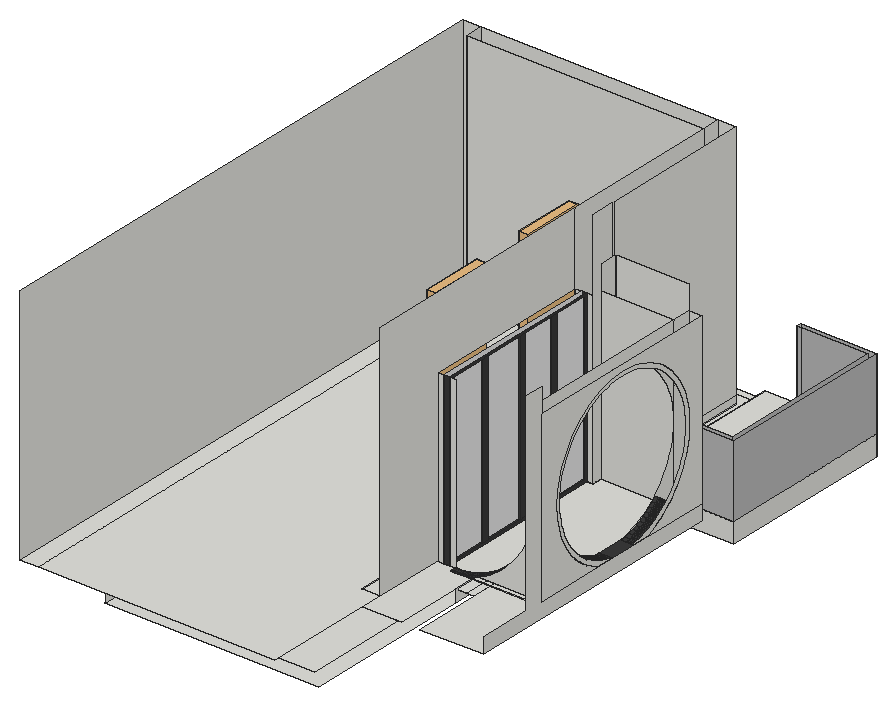
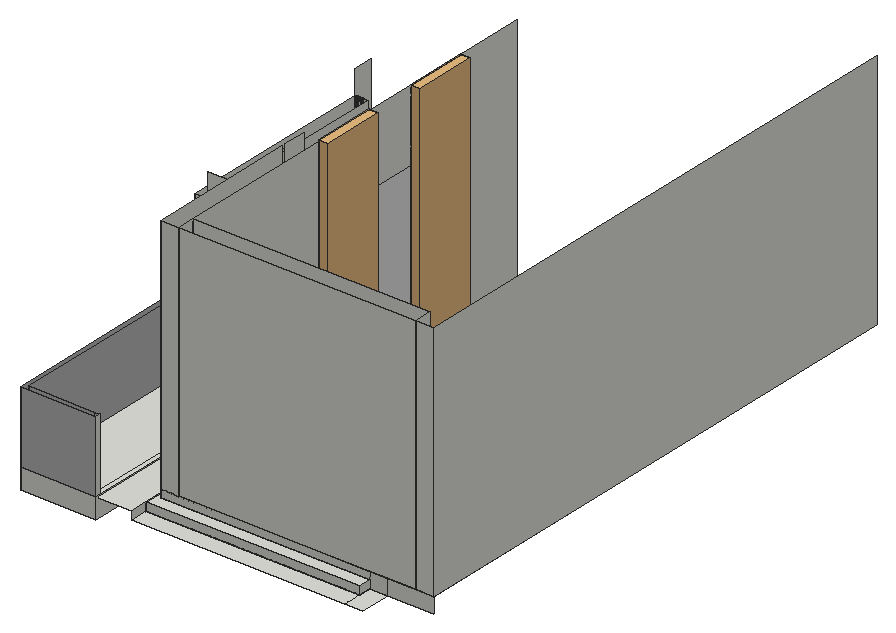
# SketchUp Ruby script. Lengths in inches.
U = 1.inch
M = Sketchup.active_model
def pt(a) = Geom::Point3d.new(a.map { |v| v * U })
def face(e, loops, mat)
  f = e.add_face(loops[0].map { |a| pt(a) })
  loops[1..].each { |l| e.add_face(l.map { |a| pt(a) }).erase! }
  f.material = f.back_material = mat if mat
  f
end
# faces: each face lists its corners as indices into pts; further lists are holes
def faces(e, pts, list, mat = nil) = list.each { |f| face(e, (f[0].is_a?(Array) ? f : [f]).map { |l| l.map { |i| pts[i] } }, mat) }
# xy, xz, yz: faces in a plane at the given z, y or x. An outline is a flat list of corners, or four numbers for a rectangle; further outlines are holes
def ring(l) = l.size == 4 ? [[l[0], l[1]], [l[2], l[1]], [l[2], l[3]], [l[0], l[3]]] : l.each_slice(2).to_a
def flat(e, list, mat, &to3) = list.each { |f| face(e, (f[0].is_a?(Array) ? f : [f]).map { |l| ring(l).map { |u, v| to3.(u, v) } }, mat) }
def xy(e, z, list, mat = nil) = flat(e, list, mat) { |x, y| [x, y, z] }
def xz(e, y, list, mat = nil) = flat(e, list, mat) { |x, z| [x, y, z] }
def yz(e, x, list, mat = nil) = flat(e, list, mat) { |y, z| [x, y, z] }
def lines(e, pts, list) = list.each { |a, b| e.add_line(pt(pts[a]), pt(pts[b])) }
# prism: a flat outline (further loops are holes) pulled along v
def prism(e, loops, v, mat = nil)
  f = face(e, loops, mat); d = Geom::Vector3d.new(v.map { |x| x * U })
  f.pushpull(f.normal.samedirection?(d) ? d.length : -d.length)
end
def box(e, o, s, mat = nil) = prism(e, [[o, [o[0] + s[0], o[1], o[2]], [o[0] + s[0], o[1] + s[1], o[2]], [o[0], o[1] + s[1], o[2]]]], [0, 0, s[2]], mat)
def at(x, y, z, deg = 0) = Geom::Transformation.translation(pt([x, y, z])) * Geom::Transformation.rotation(ORIGIN, Z_AXIS, deg.degrees)
def axes(o, x, y, z) = Geom::Transformation.new([*x, 0, *y, 0, *z, 0, *pt(o).to_a, 1])
def part(name) = M.definitions.add(name)
# library, detail: a bought-in or finely detailed component or shape, given as its bounding box
def library(name, o, s) = part(name).tap { |d| box(d.entities, o, s) }
def detail(e, o, s) = box(e.add_group.entities, o, s)
def put(e, d, t, mat = nil) = e.add_instance(d, t).tap { |i| i.material = mat if mat }
def group(e, t, mat = nil) = e.add_group.tap { |g| g.transformation = t; g.material = mat if mat }.entities
root = M.entities
M.materials.add("[Color M07]").color = [58, 58, 58]
M.materials.add("[Mirror 01]").color = [185, 185, 185]
M.materials.add("[Mirror 02]").color = [229, 229, 229]
c1 = library("Curtains 004",[-15.59,-2.26,0],[31.18,4.52,116.91])
xy(root,226.7,[[169.38,258.85,169.88,287.12]],"[Color M07]")
xy(root,228.5625,[[156.63,256.99,168.07,288.98],[169.88,256.99,174.13,288.98]])
xy(root,228.5625,[[168.07,256.99,169.88,288.98]],"[Color M07]")
xy(root,239.89,[[174.13,226.42,211.95,315.2]])
xy(root,240,[[50.2,37.13,156.63,306.2]])
xy(root,243.43,[[164.38,125.2,165.63,155.73],[164.38,159.39,165.63,193.57]],"[Color M07]")
xy(root,246,[[50.2,37.13,50.2,299.8125,154.46,299.8125,154.46,210.47,136.52,210.47,136.52,88.96,154.46,88.96,154.46,37.13],[41.2,37.45,50.2,299.8125],[136.52,88.96,136.52,210.47,154.46,210.47,154.46,224.22,156.63,224.22,156.63,88.96],[165.63,88.96,165.63,196.13,174.13,196.13,174.13,224.6,197.34,224.6,197.34,88.96],[156.63,122.64,161.76,196.13],
  [156.63,122.64,165.63,196.13],[156.63,196.13,174.13,210.47],[41.2,299.8125,50.2,315.2],[50.2,306.2,156.63,315.2]])
xy(root,246,[[161.76,122.64,165.63,196.13]],"[Color M07]")
xy(root,250.0625,[[156.63,210.47,174.13,224.6],[154.46,224.22,156.63,224.6],[154.46,224.6,156.63,224.6,156.63,306.2,50.2,306.2,50.2,299.8125,154.46,299.8125],[156.63,224.6,174.13,315.2],[174.13,226.42,174.13,228.68,209.69,228.68,209.69,312.95,174.13,312.95,174.13,315.2,211.95,315.2,211.95,226.42],
  [174.13,228.68,176.39,312.95],[176.39,228.68,209.69,312.95]])
xy(root,253.6875,[[18.46,24,27.46,299.8125],[27.46,24,145.46,24,145.46,88.96,136.52,88.96,136.52,210.47,145.46,210.47,145.46,290.8125,27.46,290.8125],[136.52,88.96,145.46,210.47],[145.46,124.96,148.9,210.47],[148.9,124.96,151.47,210.47],
  [151.47,124.96,190.96,124.96,190.96,215.22,154.46,215.22,154.46,210.47,151.47,210.47],[190.96,124.96,193.21,168.98],[193.21,124.96,193.59,168.98],[193.59,124.96,193.96,168.98],[193.96,124.96,194.34,168.98],
  [194.34,124.96,194.71,168.98],[194.71,124.96,195.09,168.98],[195.09,124.96,195.46,168.98],[195.46,124.96,195.84,168.98],[195.84,124.96,196.21,168.98],
  [196.21,124.96,196.59,168.98],[196.59,124.96,196.59,168.98,196.96,168.98,196.96,159.91,197.34,159.91,197.34,124.96],[196.96,159.91,197.34,168.98],[190.96,182.61,193.21,224.6],[193.21,182.61,193.59,224.6],
  [193.59,182.61,193.96,224.6],[193.96,182.61,194.34,224.6],[194.34,182.61,194.71,224.6],[194.71,182.61,195.09,224.6],[195.09,182.61,195.46,224.6],
  [195.46,182.61,195.84,224.6],[195.84,182.61,196.21,224.6],[196.21,182.61,196.59,224.6],[196.59,182.61,196.59,224.6,197.34,224.6,197.34,191.6875,196.96,191.6875,196.96,182.61],[196.96,182.61,197.34,191.6875],
  [145.46,210.47,154.46,299.8125],[27.46,290.8125,145.46,299.8125]])
xy(root,253.6875,[[190.96,168.98,197.34,182.61]],"[Color M07]")
xy(root,254.65,[[150.22,125.93,151.47,146.03],[150.22,149.02,151.47,169.15],[150.22,172.14,151.47,188.97],[150.22,191.96,151.47,209.51]],"[Color M07]")
xz(root,124.96,[[145.46,253.6875,148.9,337.6875],[151.47,253.6875,154.46,337.6875],[154.46,253.6875,155.66,253.71,156.86,253.76,158.0625,253.86,159.26,253.99,160.45,254.16,161.63,254.37,162.8125,254.61,163.98,254.89,165.14,255.21,166.29,255.5625,167.43,255.95,168.55,256.375,169.66,256.84,170.76,257.33,171.84,257.86,172.9,258.42,173.95,259.02,174.97,259.65,175.98,260.31,176.96,261,177.92,261.72,178.86,262.47,179.78,263.25,180.67,264.0625,181.53,264.9,182.37,265.76,183.18,266.65,183.96,267.57,184.71,268.51,185.43,269.47,186.12,270.45,186.78,271.46,187.41,272.48,188.01,273.53,188.57,274.59,189.1,275.67,189.59,276.77,190.05,277.875,190.48,279,190.87,280.14,190.96,280.4375,190.96,253.6875],[190.96,253.6875,190.96,280.4375,191.22,281.29,191.54,282.45,191.82,283.62,192.0625,284.8,192.27,285.98,192.44,287.17,192.57,288.37,192.67,289.57,192.72,290.77,192.74,291.97,192.72,293.17,192.67,294.37,192.57,295.57,192.44,296.77,192.27,297.96,192.0625,299.14,191.82,300.32,191.54,301.49,191.22,302.65,190.96,303.5,190.96,337.6875,193.21,337.6875,193.21,253.6875],[193.21,253.6875,193.59,337.6875],
  [193.59,253.6875,193.96,337.6875],[193.96,253.6875,194.34,337.6875],[194.34,253.6875,194.71,337.6875],[194.71,253.6875,195.09,337.6875],[195.09,253.6875,195.46,337.6875],
  [195.46,253.6875,195.84,337.6875],[195.84,253.6875,196.21,337.6875],[196.21,253.6875,196.59,337.6875],[196.59,253.6875,197.34,337.6875]])
xz(root,124.96,[[148.9,253.6875,151.47,337.6875]],"[Color M07]")
xz(root,125.93,[[150.22,254.65,151.47,336.73]],"[Color M07]")
xz(root,146.03,[[150.22,254.65,151.47,336.73]],"[Color M07]")
xz(root,149.02,[[150.22,254.65,151.47,336.73]],"[Color M07]")
xz(root,169.15,[[150.22,254.65,151.47,336.73]],"[Color M07]")
xz(root,172.14,[[150.22,254.65,151.47,336.73]],"[Color M07]")
xz(root,188.97,[[150.22,254.65,151.47,336.73]],"[Color M07]")
xz(root,191.96,[[150.22,254.65,151.47,336.73]],"[Color M07]")
xz(root,209.51,[[150.22,254.65,151.47,336.73]],"[Color M07]")
xz(root,210.47,[[136.52,246,154.46,253.6875],[156.63,246,174.13,250.0625],[145.46,253.6875,148.9,337.6875],[151.47,253.6875,154.46,337.6875]])
xz(root,210.47,[[148.9,253.6875,151.47,337.6875]],"[Color M07]")
xz(root,215.22,[[154.46,253.6875,190.96,337.6875]])
xz(root,224.22,[[154.46,246,156.63,250.0625]])
xz(root,224.6,[[174.13,246,174.13,250.0625,154.46,250.0625,154.46,349.6875,190.96,349.6875,190.96,253.6875,197.34,253.6875,197.34,246],[190.96,253.6875,197.34,337.6875]])
xz(root,226.42,[[174.13,239.89,211.95,250.0625]])
xz(root,226.42,[[174.13,250.0625,211.95,286.0625]],"[Mirror 01]")
xz(root,228.68,[[174.13,250.0625,176.39,286.0625]])
xz(root,228.68,[[176.39,250.0625,209.69,286.0625]],"[Mirror 01]")
xz(root,290.8125,[[27.46,253.6875,145.46,373.6875]])
xz(root,299.8125,[[18.46,246,41.2,253.6875],[41.2,246,50.2,253.6875],[50.2,246,154.46,250.0625],[50.2,250.0625,154.46,253.6875],[18.46,253.6875,27.46,373.6875],
  [27.46,253.6875,145.46,373.6875],[145.46,253.6875,154.46,373.6875]])
xz(root,306.2,[[50.2,240,156.63,246],[50.2,246,156.63,250.0625]])
xz(root,312.95,[[174.13,250.0625,176.39,286.0625],[176.39,250.0625,209.69,286.0625]],"[Mirror 01]")
xz(root,315.2,[[174.13,239.89,211.95,250.0625]])
xz(root,315.2,[[174.13,250.0625,211.95,286.0625]],"[Mirror 01]")
yz(root,18.46,[[24,253.6875,299.8125,373.6875]])
yz(root,27.46,[[290.8125,253.6875,299.8125,373.6875]])
yz(root,50.2,[[37.45,240,306.2,246],[299.8125,246,306.2,250.0625]])
yz(root,136.52,[[88.96,246,210.47,253.6875]])
yz(root,145.46,[[88.96,253.6875,88.96,373.6875,210.47,373.6875,210.47,337.6875,124.96,337.6875,124.96,253.6875],[210.47,253.6875,290.8125,373.6875],[290.8125,253.6875,299.8125,373.6875]])
yz(root,148.9,[[124.96,253.6875,210.47,337.6875]],"[Mirror 02]")
yz(root,150.22,[[125.93,254.65,146.03,336.73],[149.02,254.65,169.15,336.73],[172.14,254.65,188.97,336.73],[191.96,254.65,209.51,336.73]],"[Mirror 02]")
yz(root,151.47,[[[124.96,253.6875,210.47,337.6875],[125.93,254.65,209.51,336.73]],[146.03,254.65,149.02,336.73],[169.15,254.65,172.14,336.73],[188.97,254.65,191.96,336.73]],"[Color M07]")
yz(root,154.46,[[210.47,246,224.22,246,224.22,250.0625,224.6,250.0625,224.6,253.6875,210.47,253.6875],[224.22,246,299.8125,250.0625],[224.6,250.0625,299.8125,253.6875],[210.47,253.6875,215.22,253.6875,215.22,349.6875,222.44,349.6875,222.44,373.6875,210.47,373.6875],[215.22,253.6875,224.6,349.6875],
  [224.6,253.6875,299.8125,253.6875,299.8125,373.6875,224.22,373.6875,224.22,349.6875,224.6,349.6875]])
yz(root,156.63,[[122.64,240,196.13,246],[196.13,240,196.13,246,224.22,246,224.22,250.0625,306.2,250.0625,306.2,240],[210.47,246,224.22,250.0625],[306.2,246,315.2,250.0625]])
yz(root,174.13,[[226.42,239.89,315.2,250.0625],[210.47,246,224.6,250.0625],[226.42,250.0625,228.68,286.0625],[312.95,250.0625,315.2,286.0625]])
yz(root,190.96,[[124.96,253.6875,124.96,337.6875,215.22,337.6875,215.22,294.41,215.13,296,214.86,298.33,214.45,300.63,213.9,302.91,213.22,305.15,212.41,307.35,211.47,309.5,210.4,311.59,209.22,313.61,207.91,315.55,206.49,317.42,204.96,319.19,203.33,320.88,201.6,322.46,199.79,323.9375,197.88,325.31,195.9,326.56,193.85,327.69,191.74,328.7,189.5625,329.58,187.34,330.34,185.08,330.95,182.79,331.4375,180.47,331.78,178.14,331.99,175.8,332.0625,173.45,331.99,171.12,331.78,168.8,331.4375,166.51,330.95,164.25,330.34,162.03,329.58,159.86,328.7,157.74,327.69,155.69,326.56,153.71,325.31,151.81,323.9375,149.99,322.46,148.26,320.88,146.63,319.19,145.1,317.42,143.68,315.55,142.38,313.61,141.1875,311.59,140.12,309.5,139.18,307.35,138.37,305.15,137.6875,302.91,137.14,300.63,136.73,298.33,136.46,296,136.33,293.66,136.33,291.31,136.48,288.98,136.76,286.65,137.18,284.34,137.74,282.07,138.43,279.83,139.25,277.63,140.2,275.49,141.28,273.41,142.48,271.4,143.79,269.46,145.22,267.6,146.76,265.83,148.39,264.15,150.13,262.58,151.95,261.11,153.86,259.75,155.85,258.5,157.91,257.38,160.03,256.38,162.2,255.51,164.43,254.77,166.6875,254.16,168.98,253.6875],[182.61,253.6875,184.9,254.16,187.17,254.77,189.39,255.51,191.57,256.38,193.6875,257.38,195.74,258.5,197.73,259.75,199.64,261.11,201.46,262.58,203.2,264.15,204.84,265.83,206.37,267.6,207.8,269.46,209.12,271.4,210.3125,273.41,211.39,275.49,212.34,277.63,213.16,279.83,213.85,282.07,214.41,284.34,214.83,286.65,215.12,288.98,215.22,290.71,215.22,253.6875],[215.22,253.6875,224.6,253.6875,224.6,337.6875,215.22,337.6875,215.22,294.41,215.27,293.66,215.26,291.31,215.22,290.71]])
yz(root,196.96,[[159.91,253.6875,168.98,253.6875,166.6875,254.16,164.43,254.77,162.2,255.51,160.03,256.38,157.91,257.38,155.85,258.5,153.86,259.75,151.95,261.11,150.13,262.58,148.39,264.15,146.76,265.83,145.22,267.6,143.79,269.46,142.48,271.4,141.28,273.41,140.2,275.49,139.25,277.63,138.43,279.83,137.74,282.07,137.18,284.34,136.76,286.65,136.48,288.98,136.33,291.31,136.33,293.66,136.46,296,136.73,298.33,137.14,300.63,137.6875,302.91,138.37,305.15,139.18,307.35,140.12,309.5,141.1875,311.59,142.38,313.61,143.68,315.55,145.1,317.42,146.63,319.19,148.26,320.88,149.99,322.46,151.81,323.9375,153.71,325.31,155.69,326.56,157.74,327.69,159.86,328.7,162.03,329.58,164.25,330.34,166.51,330.95,168.8,331.4375,171.12,331.78,173.45,331.99,175.8,332.0625,178.14,331.99,180.47,331.78,182.79,331.4375,185.08,330.95,187.34,330.34,189.5625,329.58,191.74,328.7,193.85,327.69,195.9,326.56,197.88,325.31,199.79,323.9375,201.6,322.46,203.33,320.88,204.96,319.19,206.49,317.42,207.91,315.55,209.22,313.61,210.4,311.59,211.47,309.5,212.41,307.35,213.22,305.15,213.9,302.91,214.45,300.63,214.86,298.33,215.13,296,215.27,293.66,215.26,291.31,215.12,288.98,214.83,286.65,214.41,284.34,213.85,282.07,213.16,279.83,212.34,277.63,211.39,275.49,210.3125,273.41,209.12,271.4,207.8,269.46,206.37,267.6,204.84,265.83,203.2,264.15,201.46,262.58,199.64,261.11,197.73,259.75,195.74,258.5,193.6875,257.38,191.57,256.38,189.39,255.51,187.17,254.77,184.9,254.16,182.61,253.6875,191.6875,253.6875,195.87,255.97,196.9,256.53,199,257.85,201.02,259.29,202.95,260.84,204.78,262.51,206.52,264.28,208.14,266.15,209.65,268.12,211.04,270.17,212.3125,272.3,213.45,274.5,214.46,276.77,215.33,279.09,216.06,281.46,216.65,283.87,217.09,286.31,217.39,288.77,217.54,291.24,217.55,293.72,217.41,296.2,217.12,298.66,216.69,301.1,216.11,303.51,215.39,305.88,214.53,308.21,213.53,310.48,212.41,312.6875,211.15,314.82,209.77,316.88,208.26,318.85,206.65,320.73,204.92,322.51,203.1,324.1875,201.17,325.75,199.16,327.2,197.06,328.53,194.89,329.72,192.66,330.79,190.36,331.72,188.01,332.52,185.62,333.17,183.2,333.6875,180.74,334.05,178.27,334.27,175.8,334.35,173.32,334.27,170.85,334.05,168.4,333.6875,165.97,333.17,163.58,332.52,161.23,331.72,158.94,330.79,156.7,329.72,154.53,328.53,152.43,327.2,150.42,325.75,148.5,324.1875,146.67,322.51,144.94,320.73,143.33,318.85,141.83,316.88,140.44,314.82,139.1875,312.6875,138.06,310.48,137.0625,308.21,136.2,305.88,135.48,303.51,134.91,301.1,134.47,298.66,134.1875,296.2,134.04,293.72,134.05,291.24,134.2,288.77,134.5,286.31,134.95,283.87,135.54,281.46,136.27,279.09,137.14,276.77,138.14,274.5,139.28,272.3,140.55,270.17,141.94,268.12,143.45,266.15,145.08,264.28,146.81,262.51,148.64,260.84,150.58,259.29,152.59,257.85,154.7,256.53,155.73,255.97]])
yz(root,197.34,[[88.96,246,224.6,246,224.6,253.6875,124.96,253.6875,124.96,349.6875,115.33,349.6875,115.33,253.6875,88.96,253.6875],[124.96,253.6875,159.91,253.6875,155.73,255.97,154.7,256.53,152.59,257.85,150.58,259.29,148.64,260.84,146.81,262.51,145.08,264.28,143.45,266.15,141.94,268.12,140.55,270.17,139.28,272.3,138.14,274.5,137.14,276.77,136.27,279.09,135.54,281.46,134.95,283.87,134.5,286.31,134.2,288.77,134.05,291.24,134.04,293.72,134.1875,296.2,134.47,298.66,134.91,301.1,135.48,303.51,136.2,305.88,137.0625,308.21,138.06,310.48,139.1875,312.6875,140.44,314.82,141.83,316.88,143.33,318.85,144.94,320.73,146.67,322.51,148.5,324.1875,150.42,325.75,152.43,327.2,154.53,328.53,156.7,329.72,158.94,330.79,161.23,331.72,163.58,332.52,165.97,333.17,168.4,333.6875,170.85,334.05,173.32,334.27,175.8,334.35,178.27,334.27,180.74,334.05,183.2,333.6875,185.62,333.17,188.01,332.52,190.36,331.72,192.66,330.79,194.89,329.72,197.06,328.53,199.16,327.2,201.17,325.75,203.1,324.1875,204.92,322.51,206.65,320.73,208.26,318.85,209.77,316.88,211.15,314.82,212.41,312.6875,213.53,310.48,214.53,308.21,215.39,305.88,216.11,303.51,216.69,301.1,217.12,298.66,217.41,296.2,217.55,293.72,217.54,291.24,217.39,288.77,217.09,286.31,216.65,283.87,216.06,281.46,215.33,279.09,214.46,276.77,213.45,274.5,212.3125,272.3,211.04,270.17,209.65,268.12,208.14,266.15,206.52,264.28,204.78,262.51,202.95,260.84,201.02,259.29,199,257.85,196.9,256.53,195.87,255.97,191.6875,253.6875,224.6,253.6875,224.6,337.6875,124.96,337.6875]])
yz(root,209.69,[[228.68,250.0625,312.95,286.0625]],"[Mirror 01]")
yz(root,211.95,[[226.42,239.89,315.2,250.0625]])
yz(root,211.95,[[226.42,250.0625,315.2,286.0625]],"[Mirror 01]")
p = [[155.66,121.89,253.71],[155.66,122.58,253.71],[154.46,122.58,253.6875],[154.46,121.89,253.6875],[156.86,121.89,253.76],[156.86,122.58,253.76],
  [154.46,124.96,253.6875],[155.66,124.96,253.71],[156.86,124.96,253.76],[196.96,159.91,253.6875],[196.96,155.73,255.97],[197.34,155.73,255.97],
  [197.34,159.91,253.6875],[190.96,166.6875,254.16],[193.21,166.6875,254.16],[193.21,168.98,253.6875],[190.96,168.98,253.6875],[193.59,168.98,253.6875],
  [193.59,166.6875,254.16],[193.96,168.98,253.6875],[193.96,166.6875,254.16],[194.34,168.98,253.6875],[194.34,166.6875,254.16],[194.71,168.98,253.6875],
  [194.71,166.6875,254.16],[195.09,168.98,253.6875],[195.09,166.6875,254.16],[195.46,168.98,253.6875],[195.46,166.6875,254.16],[195.84,168.98,253.6875],
  [195.84,166.6875,254.16],[196.21,168.98,253.6875],[196.21,166.6875,254.16],[196.59,168.98,253.6875],[196.59,166.6875,254.16],[196.96,168.98,253.6875],
  [196.96,166.6875,254.16],[190.96,182.61,253.6875],[193.21,182.61,253.6875],[193.21,184.9,254.16],[190.96,184.9,254.16],[193.59,184.9,254.16],
  [193.59,182.61,253.6875],[193.96,184.9,254.16],[193.96,182.61,253.6875],[194.34,184.9,254.16],[194.34,182.61,253.6875],[194.71,184.9,254.16],
  [194.71,182.61,253.6875],[195.09,184.9,254.16],[195.09,182.61,253.6875],[195.46,184.9,254.16],[195.46,182.61,253.6875],[195.84,184.9,254.16],
  [195.84,182.61,253.6875],[196.21,184.9,254.16],[196.21,182.61,253.6875],[196.59,184.9,254.16],[196.59,182.61,253.6875],[196.96,184.9,254.16],
  [196.96,182.61,253.6875],[196.96,195.87,255.97],[196.96,191.6875,253.6875],[197.34,191.6875,253.6875],[197.34,195.87,255.97],[158.0625,121.89,253.86],
  [158.0625,122.58,253.86],[158.0625,124.96,253.86],[159.26,121.89,253.99],[159.26,122.58,253.99],[159.26,124.96,253.99],[160.45,121.89,254.16],
  [160.45,122.58,254.16],[160.45,124.96,254.16],[161.63,121.89,254.37],[161.63,122.58,254.37],[161.63,124.96,254.37],[190.96,164.43,254.77],
  [193.21,164.43,254.77],[193.59,164.43,254.77],[193.96,164.43,254.77],[194.34,164.43,254.77],[194.71,164.43,254.77],[195.09,164.43,254.77],
  [195.46,164.43,254.77],[195.84,164.43,254.77],[196.21,164.43,254.77],[196.59,164.43,254.77],[196.96,164.43,254.77],[193.21,187.17,254.77],
  [190.96,187.17,254.77],[193.59,187.17,254.77],[193.96,187.17,254.77],[194.34,187.17,254.77],[194.71,187.17,254.77],[195.09,187.17,254.77],
  [195.46,187.17,254.77],[195.84,187.17,254.77],[196.21,187.17,254.77],[196.59,187.17,254.77],[196.96,187.17,254.77],[162.8125,121.21,254.61],
  [162.8125,121.89,254.61],[161.63,121.21,254.37],[162.8125,122.58,254.61],[162.8125,124.96,254.61],[163.98,121.21,254.89],[163.98,121.89,254.89],
  [163.98,122.58,254.89],[163.98,124.96,254.89],[190.96,162.2,255.51],[193.21,162.2,255.51],[193.59,162.2,255.51],[193.96,162.2,255.51],
  [194.34,162.2,255.51],[194.71,162.2,255.51],[195.09,162.2,255.51],[195.46,162.2,255.51],[195.84,162.2,255.51],[196.21,162.2,255.51],
  [196.59,162.2,255.51],[196.96,162.2,255.51],[193.21,189.39,255.51],[190.96,189.39,255.51],[193.59,189.39,255.51],[193.96,189.39,255.51],
  [194.34,189.39,255.51],[194.71,189.39,255.51],[195.09,189.39,255.51],[195.46,189.39,255.51],[195.84,189.39,255.51],[196.21,189.39,255.51],
  [196.59,189.39,255.51],[196.96,189.39,255.51],[165.14,121.21,255.21],[165.14,121.89,255.21],[165.14,122.58,255.21],[165.14,124.96,255.21],
  [166.29,121.21,255.5625],[166.29,121.89,255.5625],[166.29,122.58,255.5625],[166.29,124.96,255.5625],[190.96,160.03,256.38],[193.21,160.03,256.38],
  [193.59,160.03,256.38],[193.96,160.03,256.38],[194.34,160.03,256.38],[194.71,160.03,256.38],[195.09,160.03,256.38],[195.46,160.03,256.38],
  [195.84,160.03,256.38],[196.21,160.03,256.38],[196.59,160.03,256.38],[196.96,160.03,256.38],[193.21,191.57,256.38],[190.96,191.57,256.38],
  [193.59,191.57,256.38],[193.96,191.57,256.38],[194.34,191.57,256.38],[194.71,191.57,256.38],[195.09,191.57,256.38],[195.46,191.57,256.38],
  [195.84,191.57,256.38],[196.21,191.57,256.38],[196.59,191.57,256.38],[196.96,191.57,256.38],[167.43,121.21,255.95],[167.43,121.89,255.95],
  [167.43,122.58,255.95],[167.43,124.96,255.95],[168.55,121.21,256.375],[168.55,121.89,256.375],[168.55,122.58,256.375],[168.55,124.96,256.375],
  [196.96,154.7,256.53],[197.34,154.7,256.53],[196.96,196.9,256.53],[197.34,196.9,256.53],[169.66,121.21,256.84],[169.66,121.89,256.84],
  [169.66,122.58,256.84],[169.66,124.96,256.84],[190.96,157.91,257.38],[193.21,157.91,257.38],[193.59,157.91,257.38],[193.96,157.91,257.38],
  [194.34,157.91,257.38],[194.71,157.91,257.38],[195.09,157.91,257.38],[195.46,157.91,257.38],[195.84,157.91,257.38],[196.21,157.91,257.38],
  [196.59,157.91,257.38],[196.96,157.91,257.38],[193.21,193.6875,257.38],[190.96,193.6875,257.38],[193.59,193.6875,257.38],[193.96,193.6875,257.38],
  [194.34,193.6875,257.38],[194.71,193.6875,257.38],[195.09,193.6875,257.38],[195.46,193.6875,257.38],[195.84,193.6875,257.38],[196.21,193.6875,257.38],
  [196.59,193.6875,257.38],[196.96,193.6875,257.38],[196.96,152.59,257.85],[197.34,152.59,257.85],[196.96,199,257.85],[197.34,199,257.85],
  [170.76,121.21,257.33],[170.76,121.89,257.33],[170.76,122.58,257.33],[170.76,124.96,257.33],[171.84,121.21,257.86],[171.84,121.89,257.86],
  [171.84,122.58,257.86],[171.84,124.96,257.86],[190.96,155.85,258.5],[193.21,155.85,258.5],[193.59,155.85,258.5],[193.96,155.85,258.5],
  [194.34,155.85,258.5],[194.71,155.85,258.5],[195.09,155.85,258.5],[195.46,155.85,258.5],[195.84,155.85,258.5],[196.21,155.85,258.5],
  [196.59,155.85,258.5],[196.96,155.85,258.5],[193.21,195.74,258.5],[190.96,195.74,258.5],[193.59,195.74,258.5],[193.96,195.74,258.5],
  [194.34,195.74,258.5],[194.71,195.74,258.5],[195.09,195.74,258.5],[195.46,195.74,258.5],[195.84,195.74,258.5],[196.21,195.74,258.5],
  [196.59,195.74,258.5],[196.96,195.74,258.5],[196.96,150.58,259.29],[197.34,150.58,259.29],[196.96,201.02,259.29],[197.34,201.02,259.29],
  [172.9,121.21,258.42],[172.9,121.89,258.42],[172.9,122.58,258.42],[172.9,124.96,258.42],[173.95,121.21,259.02],[173.95,121.89,259.02],
  [173.95,122.58,259.02],[173.95,124.96,259.02],[190.96,153.86,259.75],[193.21,153.86,259.75],[193.59,153.86,259.75],[193.96,153.86,259.75],
  [194.34,153.86,259.75],[194.71,153.86,259.75],[195.09,153.86,259.75],[195.46,153.86,259.75],[195.84,153.86,259.75],[196.21,153.86,259.75],
  [196.59,153.86,259.75],[196.96,153.86,259.75],[193.21,197.73,259.75],[190.96,197.73,259.75],[193.59,197.73,259.75],[193.96,197.73,259.75],
  [194.34,197.73,259.75],[194.71,197.73,259.75],[195.09,197.73,259.75],[195.46,197.73,259.75],[195.84,197.73,259.75],[196.21,197.73,259.75],
  [196.59,197.73,259.75],[196.96,197.73,259.75],[174.97,121.21,259.65],[174.97,121.89,259.65],[174.97,122.58,259.65],[174.97,124.96,259.65],
  [196.96,148.64,260.84],[197.34,148.64,260.84],[196.96,202.95,260.84],[197.34,202.95,260.84],[175.98,121.21,260.31],[175.98,121.89,260.31],
  [175.98,122.58,260.31],[175.98,124.96,260.31],[190.96,151.95,261.11],[193.21,151.95,261.11],[193.59,151.95,261.11],[193.96,151.95,261.11],
  [194.34,151.95,261.11],[194.71,151.95,261.11],[195.09,151.95,261.11],[195.46,151.95,261.11],[195.84,151.95,261.11],[196.21,151.95,261.11],
  [196.59,151.95,261.11],[196.96,151.95,261.11],[193.21,199.64,261.11],[190.96,199.64,261.11],[193.59,199.64,261.11],[193.96,199.64,261.11],
  [194.34,199.64,261.11],[194.71,199.64,261.11],[195.09,199.64,261.11],[195.46,199.64,261.11],[195.84,199.64,261.11],[196.21,199.64,261.11],
  [196.59,199.64,261.11],[196.96,199.64,261.11],[176.96,121.21,261],[176.96,121.89,261],[176.96,122.58,261],[176.96,124.96,261],
  [196.96,146.81,262.51],[197.34,146.81,262.51],[196.96,204.78,262.51],[197.34,204.78,262.51],[177.92,121.21,261.72],[177.92,121.89,261.72],
  [177.92,122.58,261.72],[177.92,124.96,261.72],[190.96,150.13,262.58],[193.21,150.13,262.58],[193.59,150.13,262.58],[193.96,150.13,262.58],
  [194.34,150.13,262.58],[194.71,150.13,262.58],[195.09,150.13,262.58],[195.46,150.13,262.58],[195.84,150.13,262.58],[196.21,150.13,262.58],
  [196.59,150.13,262.58],[196.96,150.13,262.58],[193.21,201.46,262.58],[190.96,201.46,262.58],[193.59,201.46,262.58],[193.96,201.46,262.58],
  [194.34,201.46,262.58],[194.71,201.46,262.58],[195.09,201.46,262.58],[195.46,201.46,262.58],[195.84,201.46,262.58],[196.21,201.46,262.58],
  [196.59,201.46,262.58],[196.96,201.46,262.58],[178.86,121.21,262.47],[178.86,121.89,262.47],[178.86,122.58,262.47],[178.86,124.96,262.47],
  [179.78,121.21,263.25],[179.78,121.89,263.25],[179.78,122.58,263.25],[179.78,124.96,263.25],[196.96,145.08,264.28],[197.34,145.08,264.28],
  [196.96,206.52,264.28],[197.34,206.52,264.28],[190.96,148.39,264.15],[193.21,148.39,264.15],[193.59,148.39,264.15],[193.96,148.39,264.15],
  [194.34,148.39,264.15],[194.71,148.39,264.15],[195.09,148.39,264.15],[195.46,148.39,264.15],[195.84,148.39,264.15],[196.21,148.39,264.15],
  [196.59,148.39,264.15],[196.96,148.39,264.15],[193.21,203.2,264.15],[190.96,203.2,264.15],[193.59,203.2,264.15],[193.96,203.2,264.15],
  [194.34,203.2,264.15],[194.71,203.2,264.15],[195.09,203.2,264.15],[195.46,203.2,264.15],[195.84,203.2,264.15],[196.21,203.2,264.15],
  [196.59,203.2,264.15],[196.96,203.2,264.15],[180.67,121.21,264.0625],[180.67,121.89,264.0625],[180.67,122.58,264.0625],[180.67,124.96,264.0625],
  [196.96,121.89,253.6875],[196.96,122.58,253.6875]]
faces(root,p,[[0,1,2,3],[4,5,1,0],[6,2,1,7],[7,1,5,8],[13,14,15,16],[17,15,14,18],[19,17,18,20],[21,19,20,22],
  [23,21,22,24],[25,23,24,26],[27,25,26,28],[29,27,28,30],[31,29,30,32],[33,31,32,34],[35,33,34,36],[37,38,39,40],
  [41,39,38,42],[43,41,42,44],[45,43,44,46],[47,45,46,48],[49,47,48,50],[51,49,50,52],[53,51,52,54],[55,53,54,56],
  [57,55,56,58],[59,57,58,60],[65,66,5,4],[8,5,66,67],[68,69,66,65],[67,66,69,70],[71,72,69,68],[70,69,72,73],
  [74,75,72,71],[73,72,75,76],[77,78,14,13],[18,14,78,79],[20,18,79,80],[22,20,80,81],[24,22,81,82],[26,24,82,83],
  [28,26,83,84],[30,28,84,85],[32,30,85,86],[34,32,86,87],[36,34,87,88],[40,39,89,90],[91,89,39,41],[92,91,41,43],
  [93,92,43,45],[94,93,45,47],[95,94,47,49],[96,95,49,51],[97,96,51,53],[98,97,53,55],[99,98,55,57],[100,99,57,59],
  [101,102,74,103],[102,104,75,74],[76,75,104,105],[106,107,102,101],[107,108,104,102],[105,104,108,109],[110,111,78,77],[79,78,111,112],
  [80,79,112,113],[81,80,113,114],[82,81,114,115],[83,82,115,116],[84,83,116,117],[85,84,117,118],[86,85,118,119],[87,86,119,120],
  [88,87,120,121],[90,89,122,123],[124,122,89,91],[125,124,91,92],[126,125,92,93],[127,126,93,94],[128,127,94,95],[129,128,95,96],
  [130,129,96,97],[131,130,97,98],[132,131,98,99],[133,132,99,100],[134,135,107,106],[135,136,108,107],[109,108,136,137],[138,139,135,134],
  [139,140,136,135],[137,136,140,141],[142,143,111,110],[112,111,143,144],[113,112,144,145],[114,113,145,146],[115,114,146,147],[116,115,147,148],
  [117,116,148,149],[118,117,149,150],[119,118,150,151],[120,119,151,152],[121,120,152,153],[123,122,154,155],[156,154,122,124],[157,156,124,125],
  [158,157,125,126],[159,158,126,127],[160,159,127,128],[161,160,128,129],[162,161,129,130],[163,162,130,131],[164,163,131,132],[165,164,132,133],
  [166,167,139,138],[167,168,140,139],[141,140,168,169],[170,171,167,166],[171,172,168,167],[169,168,172,173],[178,179,171,170],[179,180,172,171],
  [173,172,180,181],[182,183,143,142],[144,143,183,184],[145,144,184,185],[146,145,185,186],[147,146,186,187],[148,147,187,188],[149,148,188,189],
  [150,149,189,190],[151,150,190,191],[152,151,191,192],[153,152,192,193],[155,154,194,195],[196,194,154,156],[197,196,156,157],[198,197,157,158],
  [199,198,158,159],[200,199,159,160],[201,200,160,161],[202,201,161,162],[203,202,162,163],[204,203,163,164],[205,204,164,165],[210,211,179,178],
  [211,212,180,179],[181,180,212,213],[214,215,211,210],[215,216,212,211],[213,212,216,217],[218,219,183,182],[184,183,219,220],[185,184,220,221],
  [186,185,221,222],[187,186,222,223],[188,187,223,224],[189,188,224,225],[190,189,225,226],[191,190,226,227],[192,191,227,228],[193,192,228,229],
  [195,194,230,231],[232,230,194,196],[233,232,196,197],[234,233,197,198],[235,234,198,199],[236,235,199,200],[237,236,200,201],[238,237,201,202],
  [239,238,202,203],[240,239,203,204],[241,240,204,205],[246,247,215,214],[247,248,216,215],[217,216,248,249],[250,251,247,246],[251,252,248,247],
  [249,248,252,253],[254,255,219,218],[220,219,255,256],[221,220,256,257],[222,221,257,258],[223,222,258,259],[224,223,259,260],[225,224,260,261],
  [226,225,261,262],[227,226,262,263],[228,227,263,264],[229,228,264,265],[231,230,266,267],[268,266,230,232],[269,268,232,233],[270,269,233,234],
  [271,270,234,235],[272,271,235,236],[273,272,236,237],[274,273,237,238],[275,274,238,239],[276,275,239,240],[277,276,240,241],[278,279,251,250],
  [279,280,252,251],[253,252,280,281],[286,287,279,278],[287,288,280,279],[281,280,288,289],[290,291,255,254],[256,255,291,292],[257,256,292,293],
  [258,257,293,294],[259,258,294,295],[260,259,295,296],[261,260,296,297],[262,261,297,298],[263,262,298,299],[264,263,299,300],[265,264,300,301],
  [267,266,302,303],[304,302,266,268],[305,304,268,269],[306,305,269,270],[307,306,270,271],[308,307,271,272],[309,308,272,273],[310,309,273,274],
  [311,310,274,275],[312,311,275,276],[313,312,276,277],[314,315,287,286],[315,316,288,287],[289,288,316,317],[322,323,315,314],[323,324,316,315],
  [317,316,324,325],[326,327,291,290],[292,291,327,328],[293,292,328,329],[294,293,329,330],[295,294,330,331],[296,295,331,332],[297,296,332,333],
  [298,297,333,334],[299,298,334,335],[300,299,335,336],[301,300,336,337],[303,302,338,339],[340,338,302,304],[341,340,304,305],[342,341,305,306],
  [343,342,306,307],[344,343,307,308],[345,344,308,309],[346,345,309,310],[347,346,310,311],[348,347,311,312],[349,348,312,313],[350,351,323,322],
  [351,352,324,323],[325,324,352,353],[354,355,351,350],[355,356,352,351],[353,352,356,357],[362,363,327,326],[328,327,363,364],[329,328,364,365],
  [330,329,365,366],[331,330,366,367],[332,331,367,368],[333,332,368,369],[334,333,369,370],[335,334,370,371],[336,335,371,372],[337,336,372,373],
  [339,338,374,375],[376,374,338,340],[377,376,340,341],[378,377,341,342],[379,378,342,343],[380,379,343,344],[381,380,344,345],[382,381,345,346],
  [383,382,346,347],[384,383,347,348],[385,384,348,349],[386,387,355,354],[387,388,356,355],[357,356,388,389]],"[Color M07]")
faces(root,p,[[9,10,11,12],[61,62,63,64],[10,174,175,11],[176,61,64,177],[174,206,207,175],[208,176,177,209],[206,242,243,207],[244,208,209,245],
  [242,282,283,243],[284,244,245,285],[282,318,319,283],[320,284,285,321],[318,358,359,319],[360,320,321,361]])
lines(root,p,[[390,3],[391,2]])
put(root,c1,at(143.2,139.33,256.78,90))
put(root,c1,at(143.2,196.85,257.54,90))
